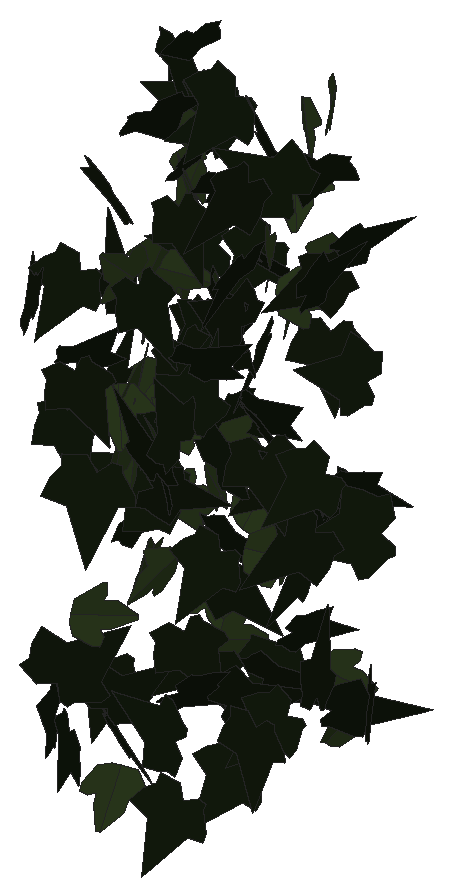
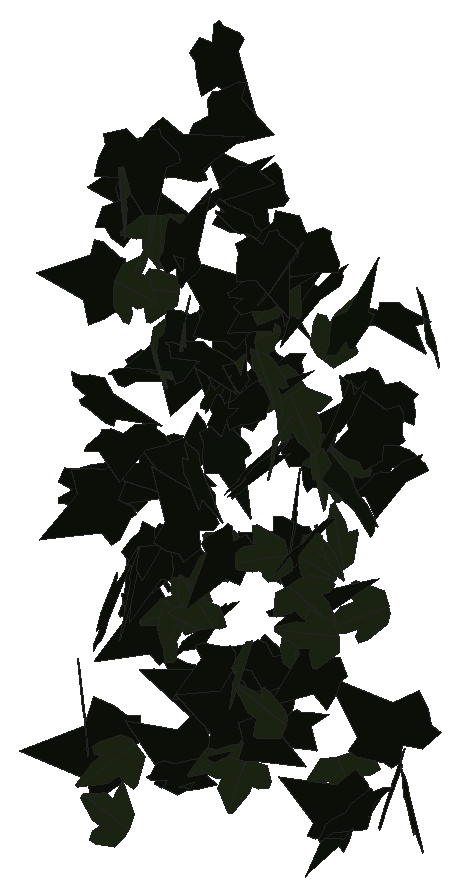
# SketchUp Ruby script. Lengths in inches.
U = 1.inch
M = Sketchup.active_model
def pt(a) = Geom::Point3d.new(a.map { |v| v * U })
def face(e, loops, mat)
  f = e.add_face(loops[0].map { |a| pt(a) })
  loops[1..].each { |l| e.add_face(l.map { |a| pt(a) }).erase! }
  f.material = f.back_material = mat if mat
  f
end
# faces: each face lists its corners as indices into pts; further lists are holes
def faces(e, pts, list, mat = nil) = list.each { |f| face(e, (f[0].is_a?(Array) ? f : [f]).map { |l| l.map { |i| pts[i] } }, mat) }
# xy, xz, yz: faces in a plane at the given z, y or x. An outline is a flat list of corners, or four numbers for a rectangle; further outlines are holes
def ring(l) = l.size == 4 ? [[l[0], l[1]], [l[2], l[1]], [l[2], l[3]], [l[0], l[3]]] : l.each_slice(2).to_a
def flat(e, list, mat, &to3) = list.each { |f| face(e, (f[0].is_a?(Array) ? f : [f]).map { |l| ring(l).map { |u, v| to3.(u, v) } }, mat) }
def xy(e, z, list, mat = nil) = flat(e, list, mat) { |x, y| [x, y, z] }
def xz(e, y, list, mat = nil) = flat(e, list, mat) { |x, z| [x, y, z] }
def yz(e, x, list, mat = nil) = flat(e, list, mat) { |y, z| [x, y, z] }
def lines(e, pts, list) = list.each { |a, b| e.add_line(pt(pts[a]), pt(pts[b])) }
# prism: a flat outline (further loops are holes) pulled along v
def prism(e, loops, v, mat = nil)
  f = face(e, loops, mat); d = Geom::Vector3d.new(v.map { |x| x * U })
  f.pushpull(f.normal.samedirection?(d) ? d.length : -d.length)
end
def box(e, o, s, mat = nil) = prism(e, [[o, [o[0] + s[0], o[1], o[2]], [o[0] + s[0], o[1] + s[1], o[2]], [o[0], o[1] + s[1], o[2]]]], [0, 0, s[2]], mat)
def at(x, y, z, deg = 0) = Geom::Transformation.translation(pt([x, y, z])) * Geom::Transformation.rotation(ORIGIN, Z_AXIS, deg.degrees)
def axes(o, x, y, z) = Geom::Transformation.new([*x, 0, *y, 0, *z, 0, *pt(o).to_a, 1])
def part(name) = M.definitions.add(name)
# library, detail: a bought-in or finely detailed component or shape, given as its bounding box
def library(name, o, s) = part(name).tap { |d| box(d.entities, o, s) }
def detail(e, o, s) = box(e.add_group.entities, o, s)
def put(e, d, t, mat = nil) = e.add_instance(d, t).tap { |i| i.material = mat if mat }
def group(e, t, mat = nil) = e.add_group.tap { |g| g.transformation = t; g.material = mat if mat }.entities
root = M.entities
M.materials.add("efeu1").color = [18, 25, 13]
M.materials.add("efeu2").color = [43, 57, 29]
c1 = part("ivyleaf_9")
p = [[1.54,2.16,1.25],[1.36,2.04,1.19],[-0.21,0.99,0.68],[-0.71,1.11,0.82],[-0.85,0.86,0.67],[-0.8,0.17,0.21],
  [-0.9,-0.01,0.1],[-0.67,-0.16,-0.02],[-0.08,-0.08,-0.05],[-0.03,-0.6,-0.4],[0.65,-0.88,-0.66],[0.83,-0.6,-0.49],
  [1.29,-0.42,-0.43],[1.8125,-0.07,-0.26],[1.21,0.44,0.15]]
faces(c1.entities,p,[[0,1,2,3,4,5,6,7,8,9,10,11,12,13,14]],"efeu1")
c2 = part("ivyleaf_10")
p = [[0,0.5,-0.03],[-0.0625,2.02,-0.43],[-0.19,2.01,-0.46],[-0.54,1.05,-0.29],[-0.52,0.625,-0.18],[-0.83,0.76,-0.28],
  [-1.16,0.64,-0.33],[-1.15,0.33,-0.24],[-0.77,-0.39,0.02],[-0.3,-0.51,0.16],[0.04,-0.48,0.23],[-0.02,2.01,-0.4375],
  [-0.06,2.01,-0.43],[0.04,-0.49,0.23],[0.67,-0.49,0.14],[1.38,0.36,-0.2],[1.375,0.51,-0.24],[0.81,0.65,-0.19],
  [0.62,0.59,-0.15],[0.6,1.09,-0.28],[0.5,1.23,-0.31]]
faces(c2.entities,p,[[0,1,2,3,4,5,6,7,8,9,10],[11,12,0,13,14,15,16,17,18,19,20]],"efeu2")
put(root,c1,axes([608.67,117.41,244.89],[-0.20717,0.08595,-1.22035],[-1.20538,0.19721,0.21852],[0.20909,1.222,0.05057]))
put(root,c2,axes([608.16,125.55,258.64],[0.79089,0.57138,-0.69021],[-0.56298,-0.39933,-0.97568],[-0.69708,0.97078,0.00489]))
put(root,c2,axes([607.33,124.78,256.34],[-0.10276,-0.02246,-1.13855],[1.1353,0.08714,-0.10418],[0.08881,-1.13985,0.01447]))
put(root,c1,axes([608.43,121.79,269.76],[0.93894,-0.92333,-0.10896],[0.07872,-0.07536,1.31687],[-0.9264,-0.94223,0.00146]))
put(root,c1,axes([609.04,121.69,264.87],[-0.24739,-0.90175,0.94208],[0.21287,0.9181,0.9347],[-1.28661,0.32529,-0.0265]))
put(root,c1,axes([608.47,121.75,245.66],[-0.22421,-1.31463,0.26561],[-0.05969,-0.25925,-1.33353],[1.33986,-0.23154,-0.01496]))
put(root,c1,axes([609.28,114.92,266.93],[-0.02859,0.3249,1.19048],[-0.22861,1.16879,-0.32447],[-1.21266,-0.228,0.03311]))
put(root,c1,axes([608.38,126.64,274.96],[0.27831,-1.01535,0.42906],[0.10196,-0.41692,-1.05275],[1.09756,0.2962,-0.011]))
put(root,c1,axes([609.34,126.54,276.08],[-0.12676,0.98364,-0.56421],[0.04554,-0.56285,-0.9915],[-1.13305,-0.13267,0.02327]))
put(root,c1,axes([609.35,122.24,253.35],[-0.14635,0.40003,-1.17061],[-0.44979,1.08089,0.4256],[1.15241,0.47268,0.01746]))
put(root,c1,axes([609.8,119.59,260.51],[-1.03774,0.99524,-0.4144],[-0.30641,0.27919,1.43782],[1.03361,1.08199,0.01017]))
put(root,c2,axes([609.7,123.82,266.62],[-0.28075,-1.09173,0.38776],[-0.11666,-0.37031,-1.12708],[1.15266,-0.30339,-0.01963]))
put(root,c2,axes([609.82,125.96,269.73],[1.08349,-0.49228,-0.32428],[-0.26701,0.1951,-1.18831],[0.52555,1.11402,0.06482]))
put(root,c1,axes([609.14,118.56,262.8125],[0.90918,0.73917,0.00032],[-0.00395,0.00435,1.17173],[0.73916,-0.90917,0.00587]))
put(root,c1,axes([609.4,117.5,260.62],[0.01253,-1.20688,-0.41496],[0.00944,0.41505,-1.20688],[1.27619,0.00878,0.013]))
put(root,c2,axes([610.65,121.76,257.72],[-0.09415,0.06695,-1.24568],[-1.01945,0.71586,0.11552],[0.71898,1.02379,0.00068]))
put(root,c2,axes([609.03,126.22,252.26],[0.39579,-0.11197,-1.11121],[1.07796,-0.27005,0.41116],[-0.29211,-1.14826,0.01166]))
put(root,c1,axes([610.66,126.17,272.91],[-0.46573,-0.90928,-0.57736],[-0.25054,-0.52031,1.02154],[-1.04755,0.52869,0.01237]))
put(root,c1,axes([610.26,117.09,268.35],[-1.09008,-0.59876,-0.10389],[0.1009,0.03205,-1.24353],[0.59927,-1.09455,0.02041]))
put(root,c1,axes([609.21,117.15,247],[-0.34223,-0.01738,1.47751],[1.47372,-0.114,0.34001],[0.10715,1.51233,0.04261]))
put(root,c2,axes([610.39,124.23,264.68],[-0.06036,0.67451,-0.93926],[-0.28549,0.90273,0.66663],[1.12057,0.26632,0.11924]))
put(root,c1,axes([610.375,122.37,274.38],[0.4833,1.3041,-0.01607],[-0.01801,-0.01047,-1.39071],[-1.30408,0.48345,0.01325]))
put(root,c1,axes([609.6,120.28,244.45],[-0.08437,-0.01502,1.26377],[1.23723,0.25767,0.08566],[-0.25809,1.2401,-0.00249]))
put(root,c1,axes([609.66,117.2,244.34],[0.35293,-0.29697,-1.23892],[1.05827,-0.64746,0.45666],[-0.70935,-1.11368,0.06487]))
put(root,c2,axes([610.08,124.49,272.99],[-1.03831,-0.09092,-0.46939],[0.46366,0.08236,-1.04159],[0.11667,-1.1365,-0.03793]))
put(root,c1,axes([611.15,122.41,255.05],[-0.5794,-1.22091,-0.61809],[-0.27982,-0.55132,1.35133],[-1.33953,0.64326,-0.01494]))
put(root,c2,axes([610.4,119.84,257.19],[0.05475,-1.16952,-0.13251],[0.01448,-0.13198,1.17077],[-1.17691,-0.05603,0.00824]))
put(root,c1,axes([610.18,119.55,244.09],[1.1127,-0.39319,-0.4114],[-0.38019,0.15867,-1.17993],[0.42344,1.17566,0.02166]))
put(root,c2,axes([610.43,120.82,258.03],[1.03643,-0.56063,0.38974],[0.34991,-0.17223,-1.17826],[0.58632,1.09381,0.01424]))
put(root,c2,axes([610.875,121.84,265.36],[0.6984,-0.97801,0.14131],[0.08231,-0.11487,-1.20178],[0.98474,0.70323,0.00022]))
put(root,c2,axes([611.56,123.86,269.52],[-0.41966,0.52817,-0.94292],[-0.67885,0.65825,0.67085],[0.84096,0.79493,0.07099]))
put(root,c1,axes([610.4375,122.37,258.89],[0.2141,-1.25302,0.05679],[0.01216,-0.05554,-1.27118],[1.25425,0.21443,0.00263]))
put(root,c2,axes([611.1,125.67,254.49],[-0.51134,0.92856,0.58567],[-0.29901,0.50386,-1.05991],[-1.05633,-0.59211,0.01652]))
put(root,c2,axes([611.11,119.7,267.43],[-0.28976,-0.7793,-0.91929],[-0.33256,-0.85707,0.83138],[-1.15837,0.441,-0.00873]))
put(root,c2,axes([611.15,120.47,262.41],[0.34208,-1.17292,-0.30443],[-0.10348,0.2869,-1.22164],[1.20735,0.35691,-0.01845]))
put(root,c1,axes([611.58,125.31,266.64],[-0.12414,-0.99125,-0.70794],[0.01127,-0.71251,0.99568],[-1.21804,0.09444,0.08136]))
put(root,c1,axes([611.09,123.5,271.36],[0.43397,0.61976,0.86427],[0.28488,0.83159,-0.73938],[-1.02464,0.4937,0.16048]))
put(root,c2,axes([610.95,120.99,251.66],[0.19244,-1.06057,-0.51515],[0.20997,-0.4828,1.0724],[-1.16022,-0.26328,0.10863]))
put(root,c2,axes([611.0625,118.96,261.36],[0.96217,0.67196,0.14092],[0.11855,0.07638,-1.17357],[-0.67627,0.96943,-0.00522]))
put(root,c2,axes([611.12,125.82,248.7],[0.90771,0.77256,0.32329],[0.24478,0.2112,-1.19196],[-0.8009,0.94013,0.00211]))
put(root,c1,axes([610.98,116.03,263.85],[-0.44163,-0.49958,-1.05988],[0.68136,0.81197,-0.66664],[0.95324,-0.81184,-0.01453]))
put(root,c2,axes([611.38,122.37,266.62],[-0.39416,-0.38346,-1.015],[0.7998,0.62706,-0.54749],[0.7332,-0.89016,0.05156]))
put(root,c1,axes([611.82,124.56,262.64],[-0.40299,-0.91252,0.85826],[-0.13765,-0.86386,-0.98311],[1.24513,-0.39084,0.16909]))
put(root,c2,axes([611.25,123.3,258.37],[0.26777,0.19879,1.12627],[0.87472,0.7096,-0.33321],[-0.73679,0.91469,0.01373]))
put(root,c1,axes([612.15,124.49,262.61],[-0.51307,-0.679,1.00469],[-0.1969,-1.02979,-0.79652],[1.19653,-0.46062,0.29974]))
put(root,c1,axes([611.33,126.04,251.22],[0.59745,-0.35896,0.96597],[0.87582,-0.41151,-0.69462],[0.54303,1.05863,0.05753]))
put(root,c2,axes([612.41,120.625,252.45],[0.03925,-0.4782,1.10118],[0.09598,-1.09699,-0.4798],[1.19668,0.10367,0.00236]))
put(root,c2,axes([611.92,115.58,251.96],[0.11623,0.18846,1.23176],[0.37827,1.17339,-0.21523],[-1.18729,0.39229,0.05201]))
put(root,c1,axes([612.59,115.45,259.42],[-0.54269,-1.29529,-0.3192],[0.11777,0.29673,-1.40437],[1.32883,-0.5553,-0.00589]))
put(root,c1,axes([612.99,124.3,258.8],[0.0448,-0.12243,-1.21855],[-0.54358,1.09068,-0.12957],[1.09744,0.54523,-0.01443]))
put(root,c1,axes([613.9,123.35,274.75],[-1.06426,0.19543,0.43685],[-0.43495,0.04934,-1.0817],[-0.19963,-1.14937,0.02784]))
put(root,c1,axes([612.875,120.29,257.02],[-0.20046,0.15131,1.19058],[0.04137,-1.20548,0.16017],[1.19944,0.06686,0.19345]))
put(root,c1,axes([612.54,119.91,256.82],[0.28318,0.31598,-1.10813],[0.52939,0.97787,0.41412],[1.0235,-0.59322,0.0924]))
put(root,c2,axes([613.33,116,243.86],[0.97911,0.72115,-0.31787],[-0.25439,-0.1906,-1.21602],[-0.74591,1.01162,-0.00252]))
put(root,c1,axes([612.72,123.83,270.47],[0.73013,1.08094,-0.29484],[0.15083,0.25389,1.30432],[1.11023,-0.74536,0.0167]))
put(root,c1,axes([613.99,123.64,263.37],[-0.53643,1.08861,-0.28537],[0.12853,-0.2548,-1.2136],[-1.11803,-0.55161,-0.0026]))
put(root,c1,axes([614.12,122.12,247.89],[-0.06092,0.11601,-1.16798],[-0.18869,-1.15531,-0.10491],[-1.15846,0.18208,0.07851]))
put(root,c1,axes([614.29,117.56,259.52],[0.60179,-0.63968,1.14776],[-0.78203,0.84012,0.87825],[-1.05592,-0.98677,0.00369]))
put(root,c2,axes([613.68,123.49,257.99],[0.10657,0.62685,1.00119],[0.22069,0.97699,-0.63519],[-1.16044,0.24337,-0.02885]))
put(root,c1,axes([613.62,120.18,271.43],[0.2631,-1.12344,-0.42317],[-0.07498,0.417,-1.15365],[1.19816,0.27279,0.02073]))
put(root,c1,axes([613.5625,117.46,268.51],[0.4845,-1.14825,-0.60892],[-0.16519,0.59018,-1.24435],[1.28918,0.50716,0.0694]))
put(root,c2,axes([613.93,123.3,248.1],[-0.0158,-0.47825,-1.14349],[0.43128,1.07001,-0.45348],[1.16203,-0.40363,0.15276]))
put(root,c1,axes([614.19,123.3,276.01],[-0.56224,-1.12342,0.65958],[-0.22334,-0.62463,-1.25427],[1.28345,-0.60083,0.07068]))
put(root,c1,axes([614.52,125.27,262.75],[-0.87011,0.49645,-0.75374],[0.65496,-0.37303,-1.00177],[-0.62098,-1.08907,-0.00046]))
put(root,c1,axes([615.03,124.7,268.1],[-1.15499,-0.43278,-0.08904],[0.08743,0.02041,-1.23336],[0.43311,-1.15824,0.01153]))
put(root,c1,axes([614.52,119.32,265.05],[0.12634,-0.88792,-0.86385],[-0.15628,0.84997,-0.89651],[1.22891,0.19938,-0.0252]))
put(root,c1,axes([614.11,122.8,251.45],[-0.09918,-0.10741,-1.24219],[0.85328,0.90274,-0.14619],[0.90911,-0.85902,0.00169]))
put(root,c2,axes([614.64,124.02,254.32],[1.14561,0.00655,-0.47295],[0.46939,0.13694,1.13889],[0.05827,-1.23181,0.1241]))
put(root,c1,axes([614.64,119.37,250.27],[-0.38297,-0.55045,-1.10479],[0.63714,0.90257,-0.67055],[1.05717,-0.74336,0.00391]))
put(root,c1,axes([615.96,124.87,246.12],[-0.79443,-0.89067,-0.32702],[-0.21794,-0.24382,1.19349],[-0.92344,0.82378,-0.00034]))
put(root,c2,axes([614.46,121.95,266.33],[-0.17154,-0.02217,1.15106],[1.09948,-0.34829,0.15714],[0.34143,1.11043,0.07227]))
put(root,c1,axes([615.57,124.83,272.33],[0.73602,-0.87988,0.7248],[-0.38042,0.62372,1.14347],[-1.07462,-0.82344,0.09164]))
put(root,c1,axes([614.57,124.74,259.22],[1.09219,0.24286,-0.50673],[0.47543,0.19104,1.11629],[0.29954,-1.18877,0.07587]))
put(root,c1,axes([614.79,122.06,265.51],[-0.14802,-0.04101,1.39155],[0.67776,-1.22448,0.036],[1.21603,0.67748,0.14932]))
put(root,c2,axes([616.42,123.1,268.45],[0.0304,-0.09578,-1.24054],[-0.40601,1.17222,-0.10045],[1.17612,0.40714,-0.00262]))
put(root,c2,axes([615.74,126.68,274.42],[-0.35122,0.96883,-0.55194],[0.22566,-0.50494,-1.02992],[-1.09194,-0.41598,-0.03531]))
put(root,c1,axes([615.79,117.61,248.47],[0.78399,0.91629,0.52329],[0.31505,0.41892,-1.20553],[-1.00706,0.84438,0.03024]))
put(root,c1,axes([615.66,121.97,264.59],[-0.01643,-0.63876,0.97555],[0.25673,-0.95369,-0.62012],[1.13745,0.20603,0.15406]))
put(root,c2,axes([616.24,124.76,253.09],[-0.02423,-0.23692,-1.21513],[0.03087,-1.2151,0.2363],[-1.23762,-0.02568,0.02968]))
put(root,c1,axes([616.75,119,255.3],[-1.0785,-0.58279,-0.13758],[0.12052,0.06636,-1.22589],[0.58656,-1.08521,-0.00108]))
put(root,c1,axes([617.11,124.26,257.23],[-0.10995,0.13138,-1.23053],[-0.24581,-1.21308,-0.10755],[-1.21287,0.23395,0.13335]))
put(root,c1,axes([615.74,123.84,267.74],[1.0815,-0.25899,0.39907],[0.39577,-0.06023,-1.11163],[0.26402,1.1512,0.03162]))
put(root,c1,axes([616.6875,117.05,263.29],[-1.20359,0.50467,0.62684],[0.5796,-0.23875,1.30511],[0.55828,1.33587,-0.00355]))
put(root,c1,axes([615.76,123.74,246.48],[0.37152,-0.36796,1.12674],[1.10672,-0.31509,-0.46782],[0.42439,1.1438,0.2336]))
put(root,c1,axes([617.08,120.15,266.7],[0.12527,0.1003,1.22912],[-0.89553,-0.84197,0.15998],[0.84783,-0.90416,-0.01263]))
put(root,c1,axes([617.375,114.96,247.74],[-0.04547,-1.34799,-0.04604],[0.00113,-0.0461,1.34876],[-1.34878,0.04541,0.00268]))
put(root,c2,axes([616.41,122.45,253.72],[0.20494,0.26603,1.22549],[0.68315,1.01763,-0.33515],[-1.05161,0.71292,0.02111]))
put(root,c1,axes([617.34,115.63,244.15],[-0.67852,-1.07607,0.20661],[-0.10977,-0.17504,-1.27213],[1.09022,-0.68734,0.0005]))
put(root,c1,axes([617.34,124.17,257.04],[1.05661,0.11688,-0.56713],[-0.56455,-0.05447,-1.06304],[-0.12877,1.19796,0.007]))
put(root,c2,axes([617.15,124.29,267.1],[0.61637,-0.80048,0.75418],[0.44453,-0.60946,-1.01016],[1.00596,0.75978,-0.01572]))
put(root,c2,axes([617.77,125.98,276.18],[0.62327,-0.92235,-0.47741],[-0.12483,0.48621,-1.10233],[1.03105,0.61642,0.15513]))
put(root,c1,axes([617.43,126.3,263.64],[-0.43849,-1.07187,-0.51547],[0.19045,0.47902,-1.15808],[1.17403,-0.47804,-0.00466]))
put(root,c2,axes([617.57,123.53,273.02],[0.90645,0.85466,0.04203],[0.02602,0.03367,-1.24582],[-0.8553,0.9068,0.00665]))
put(root,c1,axes([618.03,124.54,256.23],[0.39817,-0.24707,-1.11459],[-0.95636,0.57247,-0.46855],[0.62347,1.03592,-0.0069]))
put(root,c1,axes([616.83,122.08,260.375],[0.79274,-0.75455,0.87158],[0.64526,-0.58612,-1.09432],[0.95532,1.02203,0.01589]))
put(root,c1,axes([618.12,119.02,244.76],[-0.73663,-0.95933,0.42304],[-0.23108,-0.35574,-1.20911],[1.02268,-0.77138,0.0315]))
put(root,c1,axes([616.93,119.72,247.34],[0.42526,-0.05032,1.33235],[1.33329,0.01174,-0.42512],[0.00411,1.39852,0.0515]))
put(root,c1,axes([618.97,113.46,264.45],[-1.03582,0.20998,-0.75275],[-0.75892,0.02791,1.05209],[0.18645,1.28015,0.10053]))
put(root,c1,axes([617.97,127.22,254.28],[-0.02668,-0.40595,1.35296],[-0.19478,-1.33922,-0.40567],[1.39906,-0.19419,-0.03068]))
put(root,c2,axes([618.17,125.83,243.55],[0.15112,-0.9727,0.69265],[0.12572,0.70725,0.96577],[-1.18747,-0.0489,0.1904]))
put(root,c1,axes([617.68,117.96,260.58],[-0.02859,0.04403,1.32423],[1.00199,-0.86591,0.05042],[0.8669,1.0023,-0.01461]))
put(root,c2,axes([618.11,125.48,246.93],[-0.40867,-0.55874,-0.98942],[0.78426,0.62217,-0.67528],[0.82224,-0.87113,0.15232]))
put(root,c1,axes([619.69,120.47,274.3],[-0.21965,0.13574,1.32024],[-1.32229,0.09262,-0.22952],[-0.11405,-1.33518,0.1183]))
put(root,c1,axes([619.11,118.04,275.51],[-0.12148,0.01155,-1.42463],[0.53221,-1.32592,-0.05614],[-1.32154,-0.53504,0.10835]))
put(root,c2,axes([619.22,123.99,269.52],[0.08098,-0.76268,1.01291],[0.24042,-0.98733,-0.76264],[1.24494,0.24028,0.08139]))
put(root,c1,axes([619.73,121.65,254.59],[-1.0694,0.35134,-0.41252],[0.38746,-0.14221,-1.12555],[-0.37879,-1.13735,0.01331]))
put(root,c1,axes([620.11,119.62,247.82],[-1.06149,-0.45335,0.24188],[-0.21383,-0.11504,-1.15405],[0.46723,-1.0826,0.02134]))
put(root,c2,axes([618.98,121.49,268.24],[0.18406,-0.05145,-1.16498],[1.02266,0.57386,0.13623],[0.56035,-1.03041,0.13404]))
put(root,c1,axes([620.15,121.89,275.41],[0.44176,0.97142,-0.69498],[-0.36059,-0.59796,-1.065],[-1.1387,0.56622,0.06763]))
put(root,c1,axes([619.42,121.28,251.24],[0.67699,0.66651,0.732],[0.51068,0.52458,-0.94994],[-0.84809,0.84791,0.01231]))
put(root,c1,axes([621.01,124.22,263.43],[-0.82263,0.22365,0.92477],[-0.88141,0.28117,-0.85205],[-0.35824,-1.20534,-0.02717]))
put(root,c1,axes([619.79,124.21,269.75],[0.13119,0.98824,-0.75448],[0.03217,0.75571,0.99545],[1.2429,-0.12387,0.05387]))
put(root,c1,axes([619.42,124.19,245.92],[0.84065,0.14641,1.21125],[1.17929,0.27959,-0.85226],[-0.31278,1.44763,0.0421]))
put(root,c1,axes([619.9,113.375,268.67],[1.02216,0.69503,-0.3976],[0.33167,0.21932,1.23606],[0.7288,-1.07461,-0.00488]))
put(root,c1,axes([620.57,117.67,262.48],[-0.43961,-0.94936,-0.81169],[0.32185,0.74534,-1.04607],[1.20687,-0.54457,-0.0167]))
put(root,c1,axes([620.3125,123.41,258.05],[0.99075,0.49764,0.59362],[0.53615,0.25506,-1.10865],[-0.55908,1.12646,-0.01122]))
put(root,c1,axes([620.65,116.875,248.53],[0.05091,-1.32427,0.19587],[0.00717,-0.19574,-1.32525],[1.33865,0.05142,-0.00035]))
put(root,c1,axes([621.72,119.62,257.75],[-0.04834,-0.06097,-1.38196],[0.09827,-1.37946,0.05742],[-1.37981,-0.09611,0.05251]))
put(root,c1,axes([621.02,124.45,246.1],[-0.12555,0.49559,1.14591],[0.14036,-1.13879,0.50789],[1.24057,0.179,0.05851]))
put(root,c1,axes([622.27,120.37,271.13],[-0.19505,-0.09302,-1.22697],[0.02507,-1.24233,0.0902],[-1.23024,-0.01057,0.19637]))
put(root,c1,axes([623.1875,122.41,257.15],[-0.95392,-0.32988,1.04095],[-0.98758,-0.32911,-1.00931],[0.46591,-1.37303,-0.00816]))
put(root,c1,axes([622.85,118.52,250.53],[-0.13492,-0.5884,1.22047],[0.3798,1.16091,0.60167],[-1.30058,0.40005,0.04909]))
put(root,c1,axes([623.09,118.63,261.75],[-0.87992,-0.74934,0.47252],[-0.33709,-0.33269,-1.15531],[0.81925,-0.94173,0.03215]))
put(root,c1,axes([622.53,118.37,271.08],[0.24835,0.26229,1.23927],[0.66257,1.04943,-0.35489],[-1.07962,0.70438,0.06728]))
put(root,c1,axes([623.2,112.74,275.36],[-0.59855,0.88865,-0.8294],[0.4072,-0.7245,-1.07012],[-1.14534,-0.72199,0.05298]))
